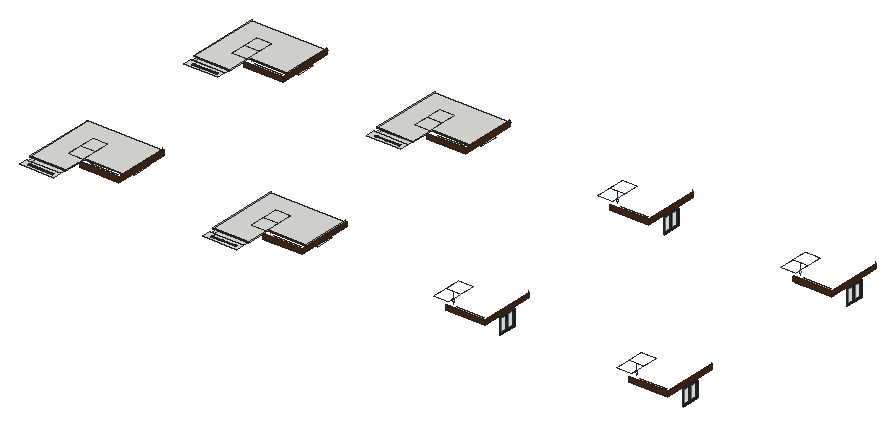
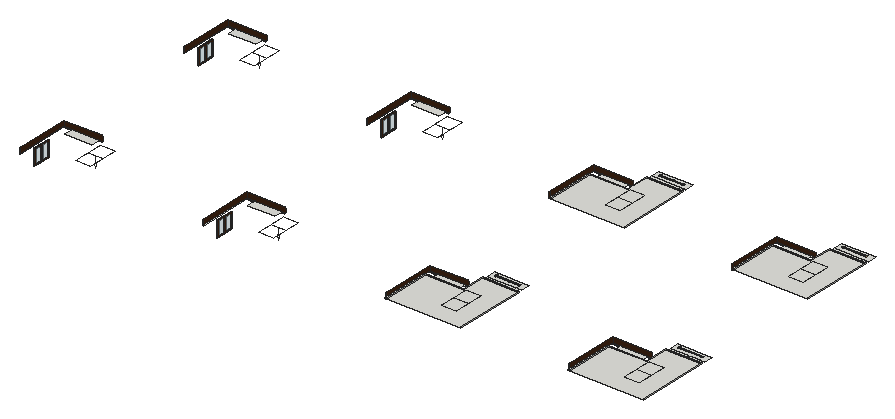
# SketchUp Ruby script. Lengths in inches.
U = 1.inch
M = Sketchup.active_model
def pt(a) = Geom::Point3d.new(a.map { |v| v * U })
def face(e, loops, mat)
  f = e.add_face(loops[0].map { |a| pt(a) })
  loops[1..].each { |l| e.add_face(l.map { |a| pt(a) }).erase! }
  f.material = f.back_material = mat if mat
  f
end
# faces: each face lists its corners as indices into pts; further lists are holes
def faces(e, pts, list, mat = nil) = list.each { |f| face(e, (f[0].is_a?(Array) ? f : [f]).map { |l| l.map { |i| pts[i] } }, mat) }
# xy, xz, yz: faces in a plane at the given z, y or x. An outline is a flat list of corners, or four numbers for a rectangle; further outlines are holes
def ring(l) = l.size == 4 ? [[l[0], l[1]], [l[2], l[1]], [l[2], l[3]], [l[0], l[3]]] : l.each_slice(2).to_a
def flat(e, list, mat, &to3) = list.each { |f| face(e, (f[0].is_a?(Array) ? f : [f]).map { |l| ring(l).map { |u, v| to3.(u, v) } }, mat) }
def xy(e, z, list, mat = nil) = flat(e, list, mat) { |x, y| [x, y, z] }
def xz(e, y, list, mat = nil) = flat(e, list, mat) { |x, z| [x, y, z] }
def yz(e, x, list, mat = nil) = flat(e, list, mat) { |y, z| [x, y, z] }
def lines(e, pts, list) = list.each { |a, b| e.add_line(pt(pts[a]), pt(pts[b])) }
# prism: a flat outline (further loops are holes) pulled along v
def prism(e, loops, v, mat = nil)
  f = face(e, loops, mat); d = Geom::Vector3d.new(v.map { |x| x * U })
  f.pushpull(f.normal.samedirection?(d) ? d.length : -d.length)
end
def box(e, o, s, mat = nil) = prism(e, [[o, [o[0] + s[0], o[1], o[2]], [o[0] + s[0], o[1] + s[1], o[2]], [o[0], o[1] + s[1], o[2]]]], [0, 0, s[2]], mat)
def at(x, y, z, deg = 0) = Geom::Transformation.translation(pt([x, y, z])) * Geom::Transformation.rotation(ORIGIN, Z_AXIS, deg.degrees)
def axes(o, x, y, z) = Geom::Transformation.new([*x, 0, *y, 0, *z, 0, *pt(o).to_a, 1])
def part(name) = M.definitions.add(name)
# library, detail: a bought-in or finely detailed component or shape, given as its bounding box
def library(name, o, s) = part(name).tap { |d| box(d.entities, o, s) }
def detail(e, o, s) = box(e.add_group.entities, o, s)
def put(e, d, t, mat = nil) = e.add_instance(d, t).tap { |i| i.material = mat if mat }
def group(e, t, mat = nil) = e.add_group.tap { |g| g.transformation = t; g.material = mat if mat }.entities
root = M.entities
M.materials.add("[Translucent Glass Safety]").color = [204, 235, 244]
M.materials["[Translucent Glass Safety]"].alpha = 0.5
M.materials.add("[Wood Veneer 01]").color = [76, 44, 23]
M.materials.add("oak swatch").color = [40, 31, 19]
c1 = part("Group\#4")
g1 = group(c1.entities,at(0,0,0))
xy(g1,0,[[0,0,6,48]],"[Wood Veneer 01]")
xy(g1,4,[[0,4,1.8125,44],[1.8125,4,6,44]])
xy(g1,80,[[0,4,1.8125,44],[1.8125,4,6,44]])
xy(g1,84,[[0,0,6,48]],"[Wood Veneer 01]")
xz(g1,0,[[0,0,6,84]],"[Wood Veneer 01]")
xz(g1,4,[[0,4,1.8125,80],[1.8125,4,6,80]])
xz(g1,44,[[0,4,1.8125,80],[1.8125,4,6,80]])
xz(g1,48,[[0,0,6,84]],"[Wood Veneer 01]")
yz(g1,0,[[[0,0,48,84],[4,4,44,80]]],"[Wood Veneer 01]")
yz(g1,1.8125,[[4,4,44,80]],"[Translucent Glass Safety]")
yz(g1,6,[[[0,0,48,84],[4,4,44,80]]],"oak swatch")
g2 = group(c1.entities,at(0,48,0),"oak swatch")
xy(g2,0,[[0,0,6,48]],"[Wood Veneer 01]")
xy(g2,4,[[0,4,1.8125,44],[1.8125,4,6,44]])
xy(g2,80,[[0,4,1.8125,44],[1.8125,4,6,44]])
xy(g2,84,[[0,0,6,48]],"[Wood Veneer 01]")
xz(g2,0,[[0,0,6,84]],"[Wood Veneer 01]")
xz(g2,4,[[0,4,1.8125,80],[1.8125,4,6,80]])
xz(g2,44,[[0,4,1.8125,80],[1.8125,4,6,80]])
xz(g2,48,[[0,0,6,84]],"[Wood Veneer 01]")
yz(g2,0,[[[0,0,48,84],[4,4,44,80]]],"[Wood Veneer 01]")
yz(g2,1.8125,[[4,4,44,80]],"[Translucent Glass Safety]")
yz(g2,6,[[[0,0,48,84],[4,4,44,80]]],"oak swatch")
c2 = part("Group264\#1")
p = [[0,0,0],[0,0,-34.62],[-5.58,0,-34.62],[36.31,-75.77,0],[-36.31,-75.77,0],[36.31,75.77,0],
  [36.31,0,0],[-36.31,75.77,0],[5.58,0,-34.62],[-36.31,0,0],[0,0,-56.04]]
lines(c2.entities,p,[[0,1],[1,2],[3,4],[5,6],[7,5],[1,8],[9,0],[0,6],[8,10],[4,9],[6,3],[2,10],
  [9,7]])
c3 = part("Rectangle Light")
put(c3.entities,c2,at(0,0,0))
c4 = library("Group\#25",[-0.5,-0.5,-0.05],[119,6.375,0.22])
xy(root,160.58,[[2450.84,831.26,2456.54,916.82],[3343.43,831.26,3349.13,916.82],[2450.84,1830.62,2456.54,1916.18],[3343.43,1830.62,3349.13,1916.18]])
xy(root,232.14,[[665.66,833.57,671.36,919.13],[1558.25,833.57,1563.95,919.13],[665.66,1832.92,671.36,1918.48],[1558.25,1832.92,1563.95,1918.48]])
xy(root,236.83,[[2450.84,831.26,2456.54,916.82],[3343.43,831.26,3349.13,916.82],[2450.84,1830.62,2456.54,1916.18],[3343.43,1830.62,3349.13,1916.18]])
xy(root,244.75,[[484.3,731.24,502.34,738.06],[502.34,731.24,634.66,776.62],[634.66,731.24,674.49,738.06],[1376.89,731.24,1394.93,738.06],[1394.93,731.24,1527.25,776.62],
  [1527.25,731.24,1567.08,738.06],[671.36,738.06,674.49,1001.66],[1563.95,738.06,1567.08,1001.66],[484.3,1730.6,502.34,1737.41],[502.34,1730.6,634.66,1775.97],
  [634.66,1730.6,674.49,1737.41],[1376.89,1730.6,1394.93,1737.41],[1394.93,1730.6,1527.25,1775.97],[1527.25,1730.6,1567.08,1737.41],[671.36,1737.41,674.49,2001.02],
  [1563.95,1737.41,1567.08,2001.02]])
xy(root,249.4375,[[2269.48,728.9375,2287.52,735.75],[2287.52,728.9375,2419.84,774.3125],[2419.84,728.9375,2459.67,735.75],[3162.07,728.9375,3180.11,735.75],[3180.11,728.9375,3312.43,774.3125],
  [3312.43,728.9375,3352.26,735.75],[2456.54,735.75,2459.67,999.35],[3349.13,735.75,3352.26,999.35],[2269.48,1728.29,2287.52,1735.1],[2287.52,1728.29,2419.84,1773.67],
  [2419.84,1728.29,2459.67,1735.1],[3162.07,1728.29,3180.11,1735.1],[3180.11,1728.29,3312.43,1773.67],[3312.43,1728.29,3352.26,1735.1],[2456.54,1735.1,2459.67,1998.71],
  [3349.13,1735.1,3352.26,1998.71]])
xy(root,252.5,[[[299.58,595.06,466.14,638.99],[331.15,611.67,331.85,611.77,332.5,612.03,333.05,612.46,333.48,613.02,333.75,613.67,333.84,614.36,333.75,615.06,333.48,615.71,333.05,616.26,332.5,616.6875,331.85,616.96,331.15,617.05,330.46,616.96,329.81,616.6875,329.25,616.26,328.83,615.71,328.56,615.06,328.47,614.36,328.56,613.67,328.83,613.02,329.25,612.46,329.81,612.03,330.46,611.77],[379.15,611.67,379.85,611.77,380.5,612.03,381.05,612.46,381.48,613.02,381.75,613.67,381.84,614.36,381.75,615.06,381.48,615.71,381.05,616.26,380.5,616.6875,379.85,616.96,379.15,617.05,378.46,616.96,377.81,616.6875,377.25,616.26,376.83,615.71,376.56,615.06,376.47,614.36,376.56,613.67,376.83,613.02,377.25,612.46,377.81,612.03,378.46,611.77],[443.78,611.67,444.47,611.77,445.12,612.03,445.68,612.46,446.11,613.02,446.375,613.67,446.47,614.36,446.375,615.06,446.11,615.71,445.68,616.26,445.12,616.6875,444.47,616.96,443.78,617.05,443.08,616.96,442.43,616.6875,441.88,616.26,441.45,615.71,441.18,615.06,441.09,614.36,441.18,613.67,441.45,613.02,441.88,612.46,442.43,612.03,443.08,611.77]],[[1192.17,595.06,1358.73,638.99],[1223.74,611.67,1224.4375,611.77,1225.09,612.03,1225.64,612.46,1226.07,613.02,1226.34,613.67,1226.43,614.36,1226.34,615.06,1226.07,615.71,1225.64,616.26,1225.09,616.6875,1224.4375,616.96,1223.74,617.05,1223.05,616.96,1222.4,616.6875,1221.84,616.26,1221.42,615.71,1221.15,615.06,1221.06,614.36,1221.15,613.67,1221.42,613.02,1221.84,612.46,1222.4,612.03,1223.05,611.77],[1271.74,611.67,1272.4375,611.77,1273.09,612.03,1273.64,612.46,1274.07,613.02,1274.34,613.67,1274.43,614.36,1274.34,615.06,1274.07,615.71,1273.64,616.26,1273.09,616.6875,1272.4375,616.96,1271.74,617.05,1271.05,616.96,1270.4,616.6875,1269.84,616.26,1269.42,615.71,1269.15,615.06,1269.06,614.36,1269.15,613.67,1269.42,613.02,1269.84,612.46,1270.4,612.03,1271.05,611.77],[1336.37,611.67,1337.0625,611.77,1337.71,612.03,1338.27,612.46,1338.7,613.02,1338.96,613.67,1339.06,614.36,1338.96,615.06,1338.7,615.71,1338.27,616.26,1337.71,616.6875,1337.0625,616.96,1336.37,617.05,1335.67,616.96,1335.02,616.6875,1334.47,616.26,1334.04,615.71,1333.77,615.06,1333.68,614.36,1333.77,613.67,1334.04,613.02,1334.47,612.46,1335.02,612.03,1335.67,611.77]],[308.96,638.99,321.33,662.52],[321.33,638.99,466.14,662.52],[1201.55,638.99,1213.92,662.52],
  [1213.92,638.99,1358.73,662.52],[[299.58,1594.41,466.14,1638.35],[331.15,1611.03,331.85,1611.12,332.5,1611.39,333.05,1611.82,333.48,1612.37,333.75,1613.02,333.84,1613.72,333.75,1614.41,333.48,1615.06,333.05,1615.62,332.5,1616.04,331.85,1616.3125,331.15,1616.4,330.46,1616.3125,329.81,1616.04,329.25,1615.62,328.83,1615.06,328.56,1614.41,328.47,1613.72,328.56,1613.02,328.83,1612.37,329.25,1611.82,329.81,1611.39,330.46,1611.12],[379.15,1611.03,379.85,1611.12,380.5,1611.39,381.05,1611.82,381.48,1612.37,381.75,1613.02,381.84,1613.72,381.75,1614.41,381.48,1615.06,381.05,1615.62,380.5,1616.04,379.85,1616.3125,379.15,1616.4,378.46,1616.3125,377.81,1616.04,377.25,1615.62,376.83,1615.06,376.56,1614.41,376.47,1613.72,376.56,1613.02,376.83,1612.37,377.25,1611.82,377.81,1611.39,378.46,1611.12],[443.78,1611.03,444.47,1611.12,445.12,1611.39,445.68,1611.82,446.11,1612.37,446.375,1613.02,446.47,1613.72,446.375,1614.41,446.11,1615.06,445.68,1615.62,445.12,1616.04,444.47,1616.3125,443.78,1616.4,443.08,1616.3125,442.43,1616.04,441.88,1615.62,441.45,1615.06,441.18,1614.41,441.09,1613.72,441.18,1613.02,441.45,1612.37,441.88,1611.82,442.43,1611.39,443.08,1611.12]],[[1192.17,1594.41,1358.73,1638.35],[1223.74,1611.03,1224.4375,1611.12,1225.09,1611.39,1225.64,1611.82,1226.07,1612.37,1226.34,1613.02,1226.43,1613.72,1226.34,1614.41,1226.07,1615.06,1225.64,1615.62,1225.09,1616.04,1224.4375,1616.3125,1223.74,1616.4,1223.05,1616.3125,1222.4,1616.04,1221.84,1615.62,1221.42,1615.06,1221.15,1614.41,1221.06,1613.72,1221.15,1613.02,1221.42,1612.37,1221.84,1611.82,1222.4,1611.39,1223.05,1611.12],[1271.74,1611.03,1272.4375,1611.12,1273.09,1611.39,1273.64,1611.82,1274.07,1612.37,1274.34,1613.02,1274.43,1613.72,1274.34,1614.41,1274.07,1615.06,1273.64,1615.62,1273.09,1616.04,1272.4375,1616.3125,1271.74,1616.4,1271.05,1616.3125,1270.4,1616.04,1269.84,1615.62,1269.42,1615.06,1269.15,1614.41,1269.06,1613.72,1269.15,1613.02,1269.42,1612.37,1269.84,1611.82,1270.4,1611.39,1271.05,1611.12],[1336.37,1611.03,1337.0625,1611.12,1337.71,1611.39,1338.27,1611.82,1338.7,1612.37,1338.96,1613.02,1339.06,1613.72,1338.96,1614.41,1338.7,1615.06,1338.27,1615.62,1337.71,1616.04,1337.0625,1616.3125,1336.37,1616.4,1335.67,1616.3125,1335.02,1616.04,1334.47,1615.62,1334.04,1615.06,1333.77,1614.41,1333.68,1613.72,1333.77,1613.02,1334.04,1612.37,1334.47,1611.82,1335.02,1611.39,1335.67,1611.12]],[308.96,1638.35,321.33,1661.875],[321.33,1638.35,466.14,1661.875],
  [1201.55,1638.35,1213.92,1661.875],[1213.92,1638.35,1358.73,1661.875]])
xy(root,254.625,[[294.47,662.52,294.47,1014.93,655.66,1014.93,655.66,776.62,471.68,776.62,471.68,662.52],[1187.0625,662.52,1187.0625,1014.93,1548.25,1014.93,1548.25,776.62,1364.27,776.62,1364.27,662.52],[655.66,776.62,665.66,1014.93],[1548.25,776.62,1558.25,1014.93],[294.47,1661.875,294.47,2014.29,655.66,2014.29,655.66,1775.97,471.68,1775.97,471.68,1661.875],
  [1187.0625,1661.875,1187.0625,2014.29,1548.25,2014.29,1548.25,1775.97,1364.27,1775.97,1364.27,1661.875],[655.66,1775.97,665.66,2014.29],[1548.25,1775.97,1558.25,2014.29]])
xz(root,662.52,[[294.47,254.625,471.68,258.1875],[1187.0625,254.625,1364.27,258.1875]])
xz(root,728.9375,[[2269.48,249.4375,2459.67,249.4375,2459.67,274.0625,2275.98,274.0625,2275.98,270.375,2269.48,270.375],[3162.07,249.4375,3352.26,249.4375,3352.26,274.0625,3168.57,274.0625,3168.57,270.375,3162.07,270.375]],"[Wood Veneer 01]")
xz(root,731.24,[[484.3,244.75,674.49,244.75,674.49,269.375,490.8,269.375,490.8,265.6875,484.3,265.6875],[1376.89,244.75,1567.08,244.75,1567.08,269.375,1383.39,269.375,1383.39,265.6875,1376.89,265.6875]],"[Wood Veneer 01]")
xz(root,776.62,[[471.68,254.625,655.66,258.1875],[1364.27,254.625,1548.25,258.1875]])
xz(root,831.26,[[2450.84,160.58,2456.54,236.83],[3343.43,160.58,3349.13,236.83]])
xz(root,916.82,[[2450.84,160.58,2456.54,236.83],[3343.43,160.58,3349.13,236.83]])
xz(root,1661.875,[[294.47,254.625,471.68,258.1875],[1187.0625,254.625,1364.27,258.1875]])
xz(root,1728.29,[[2269.48,249.4375,2459.67,249.4375,2459.67,274.0625,2275.98,274.0625,2275.98,270.375,2269.48,270.375],[3162.07,249.4375,3352.26,249.4375,3352.26,274.0625,3168.57,274.0625,3168.57,270.375,3162.07,270.375]],"[Wood Veneer 01]")
xz(root,1730.6,[[484.3,244.75,674.49,244.75,674.49,269.375,490.8,269.375,490.8,265.6875,484.3,265.6875],[1376.89,244.75,1567.08,244.75,1567.08,269.375,1383.39,269.375,1383.39,265.6875,1376.89,265.6875]],"[Wood Veneer 01]")
xz(root,1775.97,[[471.68,254.625,655.66,258.1875],[1364.27,254.625,1548.25,258.1875]])
xz(root,1830.62,[[2450.84,160.58,2456.54,236.83],[3343.43,160.58,3349.13,236.83]])
xz(root,1916.18,[[2450.84,160.58,2456.54,236.83],[3343.43,160.58,3349.13,236.83]])
yz(root,294.47,[[662.52,254.625,1014.93,258.1875],[1661.875,254.625,2014.29,258.1875]])
yz(root,471.68,[[662.52,254.625,738.06,258.1875],[738.06,254.625,776.62,258.1875],[1661.875,254.625,1737.41,258.1875],[1737.41,254.625,1775.97,258.1875]])
yz(root,655.66,[[776.62,254.625,1014.93,258.1875],[1775.97,254.625,2014.29,258.1875]])
yz(root,674.49,[[731.24,244.75,1001.66,269.375],[1730.6,244.75,2001.02,269.375]],"[Wood Veneer 01]")
yz(root,1187.0625,[[662.52,254.625,1014.93,258.1875],[1661.875,254.625,2014.29,258.1875]])
yz(root,1364.27,[[662.52,254.625,738.06,258.1875],[738.06,254.625,776.62,258.1875],[1661.875,254.625,1737.41,258.1875],[1737.41,254.625,1775.97,258.1875]])
yz(root,1548.25,[[776.62,254.625,1014.93,258.1875],[1775.97,254.625,2014.29,258.1875]])
yz(root,1567.08,[[731.24,244.75,1001.66,269.375],[1730.6,244.75,2001.02,269.375]],"[Wood Veneer 01]")
yz(root,2459.67,[[728.9375,249.4375,999.35,274.0625],[1728.29,249.4375,1998.71,274.0625]],"[Wood Veneer 01]")
yz(root,3352.26,[[728.9375,249.4375,999.35,274.0625],[1728.29,249.4375,1998.71,274.0625]],"[Wood Veneer 01]")
p = [[331.15,611.67,252.5],[330.46,611.77,252.5],[330.46,611.77,253],[331.15,611.67,253],[331.85,611.77,252.5],[331.85,611.77,253],
  [379.15,611.67,252.5],[378.46,611.77,252.5],[378.46,611.77,253.125],[379.15,611.67,253.125],[379.85,611.77,252.5],[379.85,611.77,253.125],
  [443.78,611.67,252.5],[443.08,611.77,252.5],[443.08,611.77,253.125],[443.78,611.67,253.125],[444.47,611.77,252.5],[444.47,611.77,253.125],
  [1223.74,611.67,252.5],[1223.05,611.77,252.5],[1223.05,611.77,253],[1223.74,611.67,253],[1224.4375,611.77,252.5],[1224.4375,611.77,253],
  [1271.74,611.67,252.5],[1271.05,611.77,252.5],[1271.05,611.77,253.125],[1271.74,611.67,253.125],[1272.4375,611.77,252.5],[1272.4375,611.77,253.125],
  [1336.37,611.67,252.5],[1335.67,611.77,252.5],[1335.67,611.77,253.125],[1336.37,611.67,253.125],[1337.0625,611.77,252.5],[1337.0625,611.77,253.125],
  [329.81,612.03,252.5],[329.81,612.03,253],[332.5,612.03,252.5],[332.5,612.03,253],[377.81,612.03,252.5],[377.81,612.03,253.125],
  [380.5,612.03,252.5],[380.5,612.03,253.125],[442.43,612.03,252.5],[442.43,612.03,253.125],[445.12,612.03,252.5],[445.12,612.03,253.125],
  [1222.4,612.03,252.5],[1222.4,612.03,253],[1225.09,612.03,252.5],[1225.09,612.03,253],[1270.4,612.03,252.5],[1270.4,612.03,253.125],
  [1273.09,612.03,252.5],[1273.09,612.03,253.125],[1335.02,612.03,252.5],[1335.02,612.03,253.125],[1337.71,612.03,252.5],[1337.71,612.03,253.125],
  [329.25,612.46,252.5],[329.25,612.46,253],[333.05,612.46,252.5],[333.05,612.46,253],[377.25,612.46,252.5],[377.25,612.46,253.125],
  [381.05,612.46,252.5],[381.05,612.46,253.125],[441.88,612.46,252.5],[441.88,612.46,253.125],[445.68,612.46,252.5],[445.68,612.46,253.125],
  [1221.84,612.46,252.5],[1221.84,612.46,253],[1225.64,612.46,252.5],[1225.64,612.46,253],[1269.84,612.46,252.5],[1269.84,612.46,253.125],
  [1273.64,612.46,252.5],[1273.64,612.46,253.125],[1334.47,612.46,252.5],[1334.47,612.46,253.125],[1338.27,612.46,252.5],[1338.27,612.46,253.125],
  [328.83,613.02,252.5],[328.83,613.02,253],[333.48,613.02,252.5],[333.48,613.02,253],[376.83,613.02,252.5],[376.83,613.02,253.125],
  [381.48,613.02,252.5],[381.48,613.02,253.125],[441.45,613.02,252.5],[441.45,613.02,253.125],[446.11,613.02,252.5],[446.11,613.02,253.125],
  [1221.42,613.02,252.5],[1221.42,613.02,253],[1226.07,613.02,252.5],[1226.07,613.02,253],[1269.42,613.02,252.5],[1269.42,613.02,253.125],
  [1274.07,613.02,252.5],[1274.07,613.02,253.125],[1334.04,613.02,252.5],[1334.04,613.02,253.125],[1338.7,613.02,252.5],[1338.7,613.02,253.125],
  [328.56,613.67,252.5],[328.56,613.67,253],[333.75,613.67,252.5],[333.75,613.67,253],[376.56,613.67,252.5],[376.56,613.67,253.125],
  [381.75,613.67,252.5],[381.75,613.67,253.125],[441.18,613.67,252.5],[441.18,613.67,253.125],[446.375,613.67,252.5],[446.375,613.67,253.125],
  [1221.15,613.67,252.5],[1221.15,613.67,253],[1226.34,613.67,252.5],[1226.34,613.67,253],[1269.15,613.67,252.5],[1269.15,613.67,253.125],
  [1274.34,613.67,252.5],[1274.34,613.67,253.125],[1333.77,613.67,252.5],[1333.77,613.67,253.125],[1338.96,613.67,252.5],[1338.96,613.67,253.125],
  [328.47,614.36,252.5],[328.47,614.36,253],[333.84,614.36,252.5],[333.84,614.36,253],[376.47,614.36,252.5],[376.47,614.36,253.125],
  [381.84,614.36,252.5],[381.84,614.36,253.125],[441.09,614.36,252.5],[441.09,614.36,253.125],[446.47,614.36,252.5],[446.47,614.36,253.125],
  [1221.06,614.36,252.5],[1221.06,614.36,253],[1226.43,614.36,252.5],[1226.43,614.36,253],[1269.06,614.36,252.5],[1269.06,614.36,253.125],
  [1274.43,614.36,252.5],[1274.43,614.36,253.125],[1333.68,614.36,252.5],[1333.68,614.36,253.125],[1339.06,614.36,252.5],[1339.06,614.36,253.125],
  [328.56,615.06,252.5],[328.56,615.06,253],[333.75,615.06,252.5],[333.75,615.06,253],[376.56,615.06,252.5],[376.56,615.06,253.125],
  [381.75,615.06,252.5],[381.75,615.06,253.125],[441.18,615.06,252.5],[441.18,615.06,253.125],[446.375,615.06,252.5],[446.375,615.06,253.125],
  [1221.15,615.06,252.5],[1221.15,615.06,253],[1226.34,615.06,252.5],[1226.34,615.06,253],[1269.15,615.06,252.5],[1269.15,615.06,253.125],
  [1274.34,615.06,252.5],[1274.34,615.06,253.125],[1333.77,615.06,252.5],[1333.77,615.06,253.125],[1338.96,615.06,252.5],[1338.96,615.06,253.125],
  [328.83,615.71,252.5],[328.83,615.71,253],[333.48,615.71,252.5],[333.48,615.71,253],[376.83,615.71,252.5],[376.83,615.71,253.125],
  [381.48,615.71,252.5],[381.48,615.71,253.125],[441.45,615.71,252.5],[441.45,615.71,253.125],[446.11,615.71,252.5],[446.11,615.71,253.125],
  [1221.42,615.71,252.5],[1221.42,615.71,253],[1226.07,615.71,252.5],[1226.07,615.71,253],[1269.42,615.71,252.5],[1269.42,615.71,253.125],
  [1274.07,615.71,252.5],[1274.07,615.71,253.125],[1334.04,615.71,252.5],[1334.04,615.71,253.125],[1338.7,615.71,252.5],[1338.7,615.71,253.125],
  [329.25,616.26,252.5],[329.25,616.26,253],[333.05,616.26,252.5],[333.05,616.26,253],[377.25,616.26,252.5],[377.25,616.26,253.125],
  [381.05,616.26,252.5],[381.05,616.26,253.125],[441.88,616.26,252.5],[441.88,616.26,253.125],[445.68,616.26,252.5],[445.68,616.26,253.125],
  [1221.84,616.26,252.5],[1221.84,616.26,253],[1225.64,616.26,252.5],[1225.64,616.26,253],[1269.84,616.26,252.5],[1269.84,616.26,253.125],
  [1273.64,616.26,252.5],[1273.64,616.26,253.125],[1334.47,616.26,252.5],[1334.47,616.26,253.125],[1338.27,616.26,252.5],[1338.27,616.26,253.125],
  [329.81,616.6875,252.5],[329.81,616.6875,253],[332.5,616.6875,252.5],[332.5,616.6875,253],[377.81,616.6875,252.5],[377.81,616.6875,253.125],
  [380.5,616.6875,252.5],[380.5,616.6875,253.125],[442.43,616.6875,252.5],[442.43,616.6875,253.125],[445.12,616.6875,252.5],[445.12,616.6875,253.125],
  [1222.4,616.6875,252.5],[1222.4,616.6875,253],[1225.09,616.6875,252.5],[1225.09,616.6875,253],[1270.4,616.6875,252.5],[1270.4,616.6875,253.125],
  [1273.09,616.6875,252.5],[1273.09,616.6875,253.125],[1335.02,616.6875,252.5],[1335.02,616.6875,253.125],[1337.71,616.6875,252.5],[1337.71,616.6875,253.125],
  [330.46,616.96,252.5],[330.46,616.96,253],[331.85,616.96,252.5],[331.85,616.96,253],[378.46,616.96,252.5],[378.46,616.96,253.125],
  [379.85,616.96,252.5],[379.85,616.96,253.125],[443.08,616.96,252.5],[443.08,616.96,253.125],[444.47,616.96,252.5],[444.47,616.96,253.125],
  [1223.05,616.96,252.5],[1223.05,616.96,253],[1224.4375,616.96,252.5],[1224.4375,616.96,253],[1271.05,616.96,252.5],[1271.05,616.96,253.125],
  [1272.4375,616.96,252.5],[1272.4375,616.96,253.125],[1335.67,616.96,252.5],[1335.67,616.96,253.125],[1337.0625,616.96,252.5],[1337.0625,616.96,253.125],
  [331.15,617.05,252.5],[331.15,617.05,253],[379.15,617.05,252.5],[379.15,617.05,253.125],[443.78,617.05,252.5],[443.78,617.05,253.125],
  [1223.74,617.05,252.5],[1223.74,617.05,253],[1271.74,617.05,252.5],[1271.74,617.05,253.125],[1336.37,617.05,252.5],[1336.37,617.05,253.125],
  [331.15,1611.03,252.5],[330.46,1611.12,252.5],[330.46,1611.12,253],[331.15,1611.03,253],[331.85,1611.12,252.5],[331.85,1611.12,253],
  [379.15,1611.03,252.5],[378.46,1611.12,252.5],[378.46,1611.12,253.125],[379.15,1611.03,253.125],[379.85,1611.12,252.5],[379.85,1611.12,253.125],
  [443.78,1611.03,252.5],[443.08,1611.12,252.5],[443.08,1611.12,253.125],[443.78,1611.03,253.125],[444.47,1611.12,252.5],[444.47,1611.12,253.125],
  [1223.74,1611.03,252.5],[1223.05,1611.12,252.5],[1223.05,1611.12,253],[1223.74,1611.03,253],[1224.4375,1611.12,252.5],[1224.4375,1611.12,253],
  [1271.74,1611.03,252.5],[1271.05,1611.12,252.5],[1271.05,1611.12,253.125],[1271.74,1611.03,253.125],[1272.4375,1611.12,252.5],[1272.4375,1611.12,253.125],
  [1336.37,1611.03,252.5],[1335.67,1611.12,252.5],[1335.67,1611.12,253.125],[1336.37,1611.03,253.125],[1337.0625,1611.12,252.5],[1337.0625,1611.12,253.125],
  [329.81,1611.39,252.5],[329.81,1611.39,253],[332.5,1611.39,252.5],[332.5,1611.39,253],[377.81,1611.39,252.5],[377.81,1611.39,253.125],
  [380.5,1611.39,252.5],[380.5,1611.39,253.125],[442.43,1611.39,252.5],[442.43,1611.39,253.125],[445.12,1611.39,252.5],[445.12,1611.39,253.125],
  [1222.4,1611.39,252.5],[1222.4,1611.39,253],[1225.09,1611.39,252.5],[1225.09,1611.39,253],[1270.4,1611.39,252.5],[1270.4,1611.39,253.125],
  [1273.09,1611.39,252.5],[1273.09,1611.39,253.125],[1335.02,1611.39,252.5],[1335.02,1611.39,253.125],[1337.71,1611.39,252.5],[1337.71,1611.39,253.125],
  [329.25,1611.82,252.5],[329.25,1611.82,253],[333.05,1611.82,252.5],[333.05,1611.82,253],[377.25,1611.82,252.5],[377.25,1611.82,253.125],
  [381.05,1611.82,252.5],[381.05,1611.82,253.125],[441.88,1611.82,252.5],[441.88,1611.82,253.125],[445.68,1611.82,252.5],[445.68,1611.82,253.125],
  [1221.84,1611.82,252.5],[1221.84,1611.82,253],[1225.64,1611.82,252.5],[1225.64,1611.82,253],[1269.84,1611.82,252.5],[1269.84,1611.82,253.125],
  [1273.64,1611.82,252.5],[1273.64,1611.82,253.125],[1334.47,1611.82,252.5],[1334.47,1611.82,253.125],[1338.27,1611.82,252.5],[1338.27,1611.82,253.125],
  [328.83,1612.37,252.5],[328.83,1612.37,253],[333.48,1612.37,252.5],[333.48,1612.37,253],[376.83,1612.37,252.5],[376.83,1612.37,253.125],
  [381.48,1612.37,252.5],[381.48,1612.37,253.125],[441.45,1612.37,252.5],[441.45,1612.37,253.125],[446.11,1612.37,252.5],[446.11,1612.37,253.125],
  [1221.42,1612.37,252.5],[1221.42,1612.37,253],[1226.07,1612.37,252.5],[1226.07,1612.37,253],[1269.42,1612.37,252.5],[1269.42,1612.37,253.125],
  [1274.07,1612.37,252.5],[1274.07,1612.37,253.125],[1334.04,1612.37,252.5],[1334.04,1612.37,253.125],[1338.7,1612.37,252.5],[1338.7,1612.37,253.125],
  [328.56,1613.02,252.5],[328.56,1613.02,253],[333.75,1613.02,252.5],[333.75,1613.02,253],[376.56,1613.02,252.5],[376.56,1613.02,253.125],
  [381.75,1613.02,252.5],[381.75,1613.02,253.125],[441.18,1613.02,252.5],[441.18,1613.02,253.125],[446.375,1613.02,252.5],[446.375,1613.02,253.125],
  [1221.15,1613.02,252.5],[1221.15,1613.02,253],[1226.34,1613.02,252.5],[1226.34,1613.02,253],[1269.15,1613.02,252.5],[1269.15,1613.02,253.125],
  [1274.34,1613.02,252.5],[1274.34,1613.02,253.125],[1333.77,1613.02,252.5],[1333.77,1613.02,253.125],[1338.96,1613.02,252.5],[1338.96,1613.02,253.125],
  [328.47,1613.72,252.5],[328.47,1613.72,253],[333.84,1613.72,252.5],[333.84,1613.72,253],[376.47,1613.72,252.5],[376.47,1613.72,253.125],
  [381.84,1613.72,252.5],[381.84,1613.72,253.125],[441.09,1613.72,252.5],[441.09,1613.72,253.125],[446.47,1613.72,252.5],[446.47,1613.72,253.125],
  [1221.06,1613.72,252.5],[1221.06,1613.72,253],[1226.43,1613.72,252.5],[1226.43,1613.72,253],[1269.06,1613.72,252.5],[1269.06,1613.72,253.125],
  [1274.43,1613.72,252.5],[1274.43,1613.72,253.125],[1333.68,1613.72,252.5],[1333.68,1613.72,253.125],[1339.06,1613.72,252.5],[1339.06,1613.72,253.125],
  [328.56,1614.41,252.5],[328.56,1614.41,253],[333.75,1614.41,252.5],[333.75,1614.41,253],[376.56,1614.41,252.5],[376.56,1614.41,253.125],
  [381.75,1614.41,252.5],[381.75,1614.41,253.125],[441.18,1614.41,252.5],[441.18,1614.41,253.125],[446.375,1614.41,252.5],[446.375,1614.41,253.125],
  [1221.15,1614.41,252.5],[1221.15,1614.41,253],[1226.34,1614.41,252.5],[1226.34,1614.41,253],[1269.15,1614.41,252.5],[1269.15,1614.41,253.125],
  [1274.34,1614.41,252.5],[1274.34,1614.41,253.125],[1333.77,1614.41,252.5],[1333.77,1614.41,253.125],[1338.96,1614.41,252.5],[1338.96,1614.41,253.125],
  [328.83,1615.06,252.5],[328.83,1615.06,253],[333.48,1615.06,252.5],[333.48,1615.06,253],[376.83,1615.06,252.5],[376.83,1615.06,253.125],
  [381.48,1615.06,252.5],[381.48,1615.06,253.125],[441.45,1615.06,252.5],[441.45,1615.06,253.125],[446.11,1615.06,252.5],[446.11,1615.06,253.125],
  [1221.42,1615.06,252.5],[1221.42,1615.06,253],[1226.07,1615.06,252.5],[1226.07,1615.06,253],[1269.42,1615.06,252.5],[1269.42,1615.06,253.125],
  [1274.07,1615.06,252.5],[1274.07,1615.06,253.125],[1334.04,1615.06,252.5],[1334.04,1615.06,253.125],[1338.7,1615.06,252.5],[1338.7,1615.06,253.125],
  [329.25,1615.62,252.5],[329.25,1615.62,253],[333.05,1615.62,252.5],[333.05,1615.62,253],[377.25,1615.62,252.5],[377.25,1615.62,253.125],
  [381.05,1615.62,252.5],[381.05,1615.62,253.125],[441.88,1615.62,252.5],[441.88,1615.62,253.125],[445.68,1615.62,252.5],[445.68,1615.62,253.125],
  [1221.84,1615.62,252.5],[1221.84,1615.62,253],[1225.64,1615.62,252.5],[1225.64,1615.62,253],[1269.84,1615.62,252.5],[1269.84,1615.62,253.125],
  [1273.64,1615.62,252.5],[1273.64,1615.62,253.125],[1334.47,1615.62,252.5],[1334.47,1615.62,253.125],[1338.27,1615.62,252.5],[1338.27,1615.62,253.125],
  [329.81,1616.04,252.5],[329.81,1616.04,253],[332.5,1616.04,252.5],[332.5,1616.04,253],[377.81,1616.04,252.5],[377.81,1616.04,253.125],
  [380.5,1616.04,252.5],[380.5,1616.04,253.125],[442.43,1616.04,252.5],[442.43,1616.04,253.125],[445.12,1616.04,252.5],[445.12,1616.04,253.125],
  [1222.4,1616.04,252.5],[1222.4,1616.04,253],[1225.09,1616.04,252.5],[1225.09,1616.04,253],[1270.4,1616.04,252.5],[1270.4,1616.04,253.125],
  [1273.09,1616.04,252.5],[1273.09,1616.04,253.125],[1335.02,1616.04,252.5],[1335.02,1616.04,253.125],[1337.71,1616.04,252.5],[1337.71,1616.04,253.125],
  [330.46,1616.3125,252.5],[330.46,1616.3125,253],[331.85,1616.3125,252.5],[331.85,1616.3125,253],[378.46,1616.3125,252.5],[378.46,1616.3125,253.125],
  [379.85,1616.3125,252.5],[379.85,1616.3125,253.125],[443.08,1616.3125,252.5],[443.08,1616.3125,253.125],[444.47,1616.3125,252.5],[444.47,1616.3125,253.125],
  [1223.05,1616.3125,252.5],[1223.05,1616.3125,253],[1224.4375,1616.3125,252.5],[1224.4375,1616.3125,253],[1271.05,1616.3125,252.5],[1271.05,1616.3125,253.125],
  [1272.4375,1616.3125,252.5],[1272.4375,1616.3125,253.125],[1335.67,1616.3125,252.5],[1335.67,1616.3125,253.125],[1337.0625,1616.3125,252.5],[1337.0625,1616.3125,253.125],
  [331.15,1616.4,252.5],[331.15,1616.4,253],[379.15,1616.4,252.5],[379.15,1616.4,253.125],[443.78,1616.4,252.5],[443.78,1616.4,253.125],
  [1223.74,1616.4,252.5],[1223.74,1616.4,253],[1271.74,1616.4,252.5],[1271.74,1616.4,253.125],[1336.37,1616.4,252.5],[1336.37,1616.4,253.125],
  [2456.54,999.35,249.4375],[2456.54,999.35,282.1875],[3349.13,999.35,249.4375],[3349.13,999.35,282.1875],[1563.95,1001.66,244.75],[1563.95,1001.66,277.5],
  [671.36,1001.66,244.75],[671.36,1001.66,277.5],[3349.13,1998.71,249.4375],[3349.13,1998.71,282.1875],[2456.54,1998.71,249.4375],[2456.54,1998.71,282.1875],
  [671.36,2001.02,244.75],[671.36,2001.02,277.5],[1563.95,2001.02,244.75],[1563.95,2001.02,277.5]]
faces(root,p,[[0,1,2,3],[4,0,3,5],[6,7,8,9],[10,6,9,11],[12,13,14,15],[16,12,15,17],[18,19,20,21],[22,18,21,23],
  [24,25,26,27],[28,24,27,29],[30,31,32,33],[34,30,33,35],[1,36,37,2],[38,4,5,39],[7,40,41,8],[42,10,11,43],
  [13,44,45,14],[46,16,17,47],[19,48,49,20],[50,22,23,51],[25,52,53,26],[54,28,29,55],[31,56,57,32],[58,34,35,59],
  [36,60,61,37],[62,38,39,63],[40,64,65,41],[66,42,43,67],[44,68,69,45],[70,46,47,71],[48,72,73,49],[74,50,51,75],
  [52,76,77,53],[78,54,55,79],[56,80,81,57],[82,58,59,83],[60,84,85,61],[86,62,63,87],[64,88,89,65],[90,66,67,91],
  [68,92,93,69],[94,70,71,95],[72,96,97,73],[98,74,75,99],[76,100,101,77],[102,78,79,103],[80,104,105,81],[106,82,83,107],
  [84,108,109,85],[110,86,87,111],[88,112,113,89],[114,90,91,115],[92,116,117,93],[118,94,95,119],[96,120,121,97],[122,98,99,123],
  [100,124,125,101],[126,102,103,127],[104,128,129,105],[130,106,107,131],[108,132,133,109],[134,110,111,135],[112,136,137,113],[138,114,115,139],
  [116,140,141,117],[142,118,119,143],[120,144,145,121],[146,122,123,147],[124,148,149,125],[150,126,127,151],[128,152,153,129],[154,130,131,155],
  [132,156,157,133],[158,134,135,159],[136,160,161,137],[162,138,139,163],[140,164,165,141],[166,142,143,167],[144,168,169,145],[170,146,147,171],
  [148,172,173,149],[174,150,151,175],[152,176,177,153],[178,154,155,179],[156,180,181,157],[182,158,159,183],[160,184,185,161],[186,162,163,187],
  [164,188,189,165],[190,166,167,191],[168,192,193,169],[194,170,171,195],[172,196,197,173],[198,174,175,199],[176,200,201,177],[202,178,179,203],
  [180,204,205,181],[206,182,183,207],[184,208,209,185],[210,186,187,211],[188,212,213,189],[214,190,191,215],[192,216,217,193],[218,194,195,219],
  [196,220,221,197],[222,198,199,223],[200,224,225,201],[226,202,203,227],[204,228,229,205],[230,206,207,231],[208,232,233,209],[234,210,211,235],
  [212,236,237,213],[238,214,215,239],[216,240,241,217],[242,218,219,243],[220,244,245,221],[246,222,223,247],[224,248,249,225],[250,226,227,251],
  [228,252,253,229],[254,230,231,255],[232,256,257,233],[258,234,235,259],[236,260,261,237],[262,238,239,263],[240,264,265,241],[266,242,243,267],
  [244,268,269,245],[270,246,247,271],[248,272,273,249],[274,250,251,275],[252,276,277,253],[276,254,255,277],[256,278,279,257],[278,258,259,279],
  [260,280,281,261],[280,262,263,281],[264,282,283,265],[282,266,267,283],[268,284,285,269],[284,270,271,285],[272,286,287,273],[286,274,275,287],
  [288,289,290,291],[292,288,291,293],[294,295,296,297],[298,294,297,299],[300,301,302,303],[304,300,303,305],[306,307,308,309],[310,306,309,311],
  [312,313,314,315],[316,312,315,317],[318,319,320,321],[322,318,321,323],[289,324,325,290],[326,292,293,327],[295,328,329,296],[330,298,299,331],
  [301,332,333,302],[334,304,305,335],[307,336,337,308],[338,310,311,339],[313,340,341,314],[342,316,317,343],[319,344,345,320],[346,322,323,347],
  [324,348,349,325],[350,326,327,351],[328,352,353,329],[354,330,331,355],[332,356,357,333],[358,334,335,359],[336,360,361,337],[362,338,339,363],
  [340,364,365,341],[366,342,343,367],[344,368,369,345],[370,346,347,371],[348,372,373,349],[374,350,351,375],[352,376,377,353],[378,354,355,379],
  [356,380,381,357],[382,358,359,383],[360,384,385,361],[386,362,363,387],[364,388,389,365],[390,366,367,391],[368,392,393,369],[394,370,371,395],
  [372,396,397,373],[398,374,375,399],[376,400,401,377],[402,378,379,403],[380,404,405,381],[406,382,383,407],[384,408,409,385],[410,386,387,411],
  [388,412,413,389],[414,390,391,415],[392,416,417,393],[418,394,395,419],[396,420,421,397],[422,398,399,423],[400,424,425,401],[426,402,403,427],
  [404,428,429,405],[430,406,407,431],[408,432,433,409],[434,410,411,435],[412,436,437,413],[438,414,415,439],[416,440,441,417],[442,418,419,443],
  [420,444,445,421],[446,422,423,447],[424,448,449,425],[450,426,427,451],[428,452,453,429],[454,430,431,455],[432,456,457,433],[458,434,435,459],
  [436,460,461,437],[462,438,439,463],[440,464,465,441],[466,442,443,467],[444,468,469,445],[470,446,447,471],[448,472,473,449],[474,450,451,475],
  [452,476,477,453],[478,454,455,479],[456,480,481,457],[482,458,459,483],[460,484,485,461],[486,462,463,487],[464,488,489,465],[490,466,467,491],
  [468,492,493,469],[494,470,471,495],[472,496,497,473],[498,474,475,499],[476,500,501,477],[502,478,479,503],[480,504,505,481],[506,482,483,507],
  [484,508,509,485],[510,486,487,511],[488,512,513,489],[514,490,491,515],[492,516,517,493],[518,494,495,519],[496,520,521,497],[522,498,499,523],
  [500,524,525,501],[526,502,503,527],[504,528,529,505],[530,506,507,531],[508,532,533,509],[534,510,511,535],[512,536,537,513],[538,514,515,539],
  [516,540,541,517],[542,518,519,543],[520,544,545,521],[546,522,523,547],[524,548,549,525],[550,526,527,551],[528,552,553,529],[554,530,531,555],
  [532,556,557,533],[558,534,535,559],[536,560,561,537],[562,538,539,563],[540,564,565,541],[564,542,543,565],[544,566,567,545],[566,546,547,567],
  [548,568,569,549],[568,550,551,569],[552,570,571,553],[570,554,555,571],[556,572,573,557],[572,558,559,573],[560,574,575,561],[574,562,563,575]])
lines(root,p,[[576,577],[578,579],[580,581],[582,583],[584,585],[586,587],[588,589],[590,591]])
put(root,c1,axes([2450.54,831.26,160.58],[1,0,0],[0,0.88868,0],[0,0,0.90774]))
put(root,c1,axes([2450.54,1830.62,160.58],[1,0,0],[0,0.88868,0],[0,0,0.90774]))
put(root,c1,axes([3343.13,831.26,160.58],[1,0,0],[0,0.88868,0],[0,0,0.90774]))
put(root,c1,axes([3343.13,1830.62,160.58],[1,0,0],[0,0.88868,0],[0,0,0.90774]))
put(root,c3,at(427.77,849.13,254.61))
put(root,c3,at(427.77,1848.49,254.61))
put(root,c3,at(1320.36,849.13,254.62))
put(root,c3,at(1320.36,1848.49,254.62))
put(root,c3,at(2212.95,1846.18,259.3))
put(root,c3,at(2212.95,846.83,259.3))
put(root,c3,at(3105.54,1846.18,259.3))
put(root,c3,at(3105.54,846.83,259.3))
put(root,c4,at(328.47,1611.03,253))
put(root,c4,at(328.47,611.67,253))
put(root,c4,at(1221.06,1611.03,253))
put(root,c4,at(1221.06,611.67,253))
